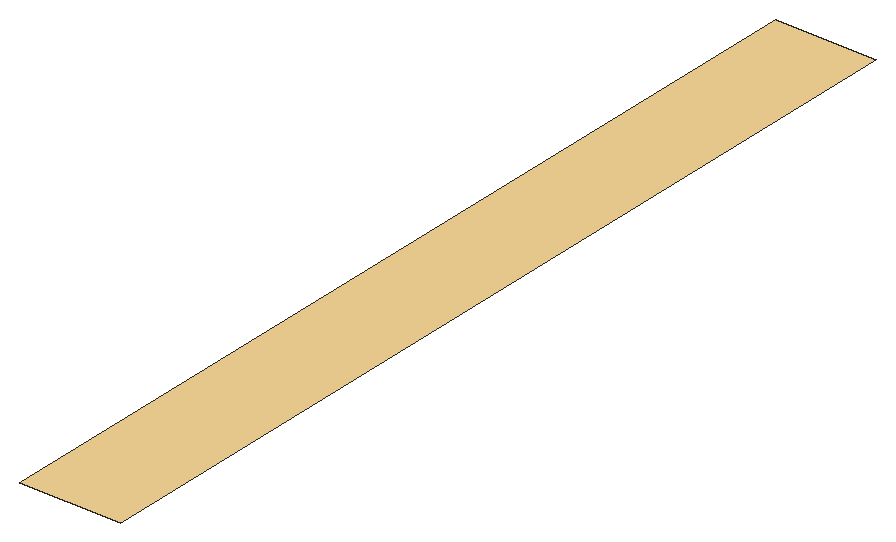
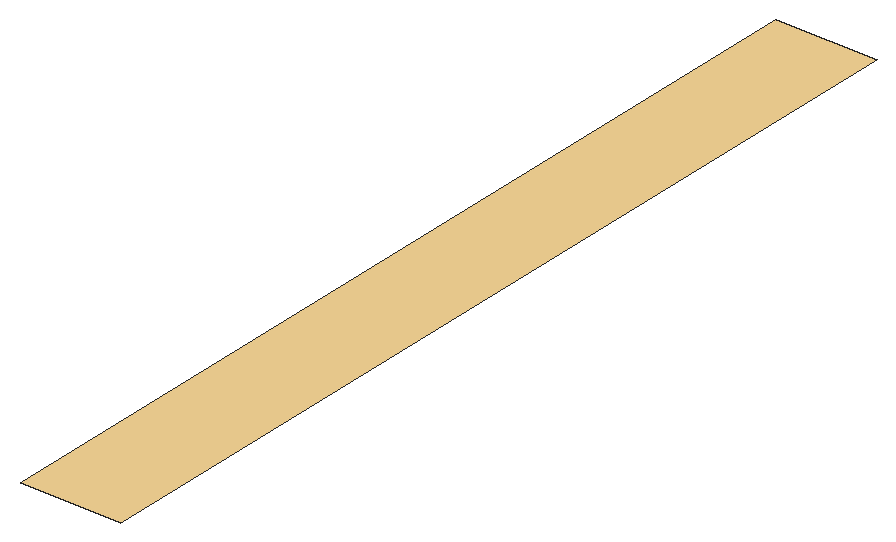
# SketchUp Ruby script. Lengths in inches.
U = 1.inch
M = Sketchup.active_model
def pt(a) = Geom::Point3d.new(a.map { |v| v * U })
def face(e, loops, mat)
  f = e.add_face(loops[0].map { |a| pt(a) })
  loops[1..].each { |l| e.add_face(l.map { |a| pt(a) }).erase! }
  f.material = f.back_material = mat if mat
  f
end
# faces: each face lists its corners as indices into pts; further lists are holes
def faces(e, pts, list, mat = nil) = list.each { |f| face(e, (f[0].is_a?(Array) ? f : [f]).map { |l| l.map { |i| pts[i] } }, mat) }
# xy, xz, yz: faces in a plane at the given z, y or x. An outline is a flat list of corners, or four numbers for a rectangle; further outlines are holes
def ring(l) = l.size == 4 ? [[l[0], l[1]], [l[2], l[1]], [l[2], l[3]], [l[0], l[3]]] : l.each_slice(2).to_a
def flat(e, list, mat, &to3) = list.each { |f| face(e, (f[0].is_a?(Array) ? f : [f]).map { |l| ring(l).map { |u, v| to3.(u, v) } }, mat) }
def xy(e, z, list, mat = nil) = flat(e, list, mat) { |x, y| [x, y, z] }
def xz(e, y, list, mat = nil) = flat(e, list, mat) { |x, z| [x, y, z] }
def yz(e, x, list, mat = nil) = flat(e, list, mat) { |y, z| [x, y, z] }
def lines(e, pts, list) = list.each { |a, b| e.add_line(pt(pts[a]), pt(pts[b])) }
# prism: a flat outline (further loops are holes) pulled along v
def prism(e, loops, v, mat = nil)
  f = face(e, loops, mat); d = Geom::Vector3d.new(v.map { |x| x * U })
  f.pushpull(f.normal.samedirection?(d) ? d.length : -d.length)
end
def box(e, o, s, mat = nil) = prism(e, [[o, [o[0] + s[0], o[1], o[2]], [o[0] + s[0], o[1] + s[1], o[2]], [o[0], o[1] + s[1], o[2]]]], [0, 0, s[2]], mat)
def at(x, y, z, deg = 0) = Geom::Transformation.translation(pt([x, y, z])) * Geom::Transformation.rotation(ORIGIN, Z_AXIS, deg.degrees)
def axes(o, x, y, z) = Geom::Transformation.new([*x, 0, *y, 0, *z, 0, *pt(o).to_a, 1])
def part(name) = M.definitions.add(name)
# library, detail: a bought-in or finely detailed component or shape, given as its bounding box
def library(name, o, s) = part(name).tap { |d| box(d.entities, o, s) }
def detail(e, o, s) = box(e.add_group.entities, o, s)
def put(e, d, t, mat = nil) = e.add_instance(d, t).tap { |i| i.material = mat if mat }
def group(e, t, mat = nil) = e.add_group.tap { |g| g.transformation = t; g.material = mat if mat }.entities
root = M.entities
M.materials.add("Outer Light").color = [251, 217, 152]
xy(root,171.29,[[278.84,95.37,279,96.87]],"Outer Light")
